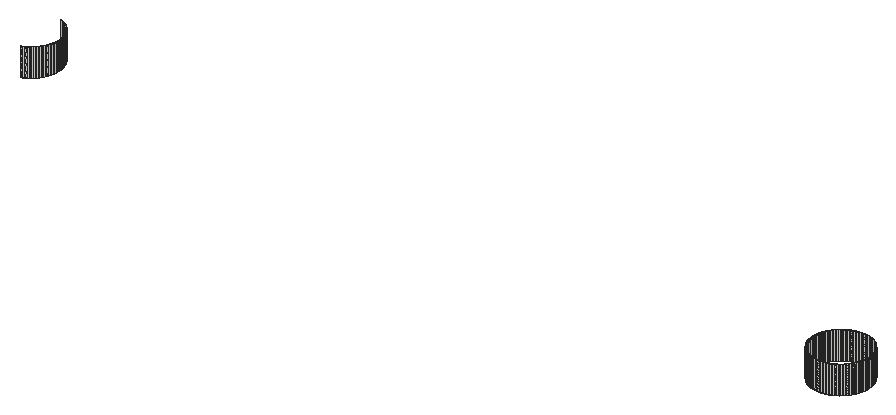
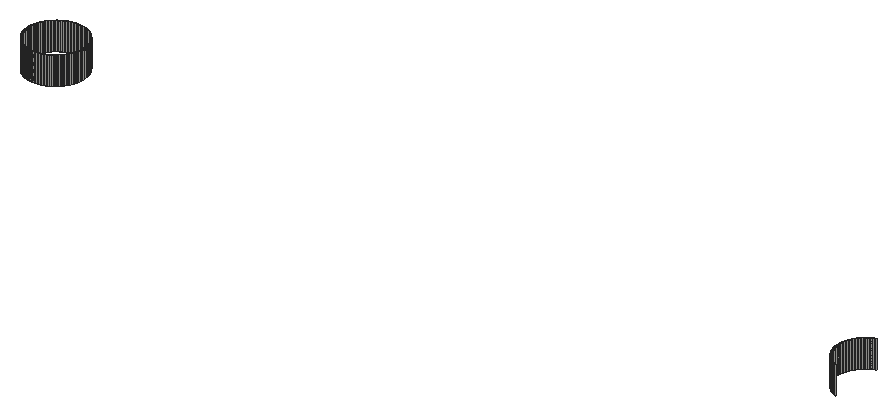
# SketchUp Ruby script. Lengths in inches.
U = 1.inch
M = Sketchup.active_model
def pt(a) = Geom::Point3d.new(a.map { |v| v * U })
def face(e, loops, mat)
  f = e.add_face(loops[0].map { |a| pt(a) })
  loops[1..].each { |l| e.add_face(l.map { |a| pt(a) }).erase! }
  f.material = f.back_material = mat if mat
  f
end
# faces: each face lists its corners as indices into pts; further lists are holes
def faces(e, pts, list, mat = nil) = list.each { |f| face(e, (f[0].is_a?(Array) ? f : [f]).map { |l| l.map { |i| pts[i] } }, mat) }
# xy, xz, yz: faces in a plane at the given z, y or x. An outline is a flat list of corners, or four numbers for a rectangle; further outlines are holes
def ring(l) = l.size == 4 ? [[l[0], l[1]], [l[2], l[1]], [l[2], l[3]], [l[0], l[3]]] : l.each_slice(2).to_a
def flat(e, list, mat, &to3) = list.each { |f| face(e, (f[0].is_a?(Array) ? f : [f]).map { |l| ring(l).map { |u, v| to3.(u, v) } }, mat) }
def xy(e, z, list, mat = nil) = flat(e, list, mat) { |x, y| [x, y, z] }
def xz(e, y, list, mat = nil) = flat(e, list, mat) { |x, z| [x, y, z] }
def yz(e, x, list, mat = nil) = flat(e, list, mat) { |y, z| [x, y, z] }
def lines(e, pts, list) = list.each { |a, b| e.add_line(pt(pts[a]), pt(pts[b])) }
# prism: a flat outline (further loops are holes) pulled along v
def prism(e, loops, v, mat = nil)
  f = face(e, loops, mat); d = Geom::Vector3d.new(v.map { |x| x * U })
  f.pushpull(f.normal.samedirection?(d) ? d.length : -d.length)
end
def box(e, o, s, mat = nil) = prism(e, [[o, [o[0] + s[0], o[1], o[2]], [o[0] + s[0], o[1] + s[1], o[2]], [o[0], o[1] + s[1], o[2]]]], [0, 0, s[2]], mat)
def at(x, y, z, deg = 0) = Geom::Transformation.translation(pt([x, y, z])) * Geom::Transformation.rotation(ORIGIN, Z_AXIS, deg.degrees)
def axes(o, x, y, z) = Geom::Transformation.new([*x, 0, *y, 0, *z, 0, *pt(o).to_a, 1])
def part(name) = M.definitions.add(name)
# library, detail: a bought-in or finely detailed component or shape, given as its bounding box
def library(name, o, s) = part(name).tap { |d| box(d.entities, o, s) }
def detail(e, o, s) = box(e.add_group.entities, o, s)
def put(e, d, t, mat = nil) = e.add_instance(d, t).tap { |i| i.material = mat if mat }
def group(e, t, mat = nil) = e.add_group.tap { |g| g.transformation = t; g.material = mat if mat }.entities
root = M.entities
xz(root,174.5,[[291.84,258,291.92,261],[291.92,258,292,261],[292,258,292.08,261],[292.08,258,292.16,261]])
xz(root,180.5,[[291.84,258,291.92,261],[291.92,258,292,261],[292,258,292.08,261],[292.08,258,292.16,261]])
yz(root,207.32,[[177.1875,258,177.26,261],[177.74,258,177.8125,261]])
yz(root,207.33,[[177.34,258,177.42,261],[177.42,258,177.5,261],[177.5,258,177.58,261],[177.58,258,177.66,261]])
yz(root,289,[[177.34,258,177.42,261],[177.42,258,177.5,261],[177.5,258,177.58,261],[177.58,258,177.66,261]])
yz(root,295,[[177.34,258,177.42,261],[177.42,258,177.5,261],[177.5,258,177.58,261],[177.58,258,177.66,261]])
p = [[291.53,174.54,258],[291.45,174.55,258],[291.45,174.55,261],[291.53,174.54,261],[291.61,174.53,258],[291.61,174.53,261],
  [291.6875,174.52,258],[291.6875,174.52,261],[291.76,174.51,258],[291.76,174.51,261],[291.84,174.5,258],[291.84,174.5,261],
  [292.24,174.51,258],[292.16,174.5,258],[292.16,174.5,261],[292.24,174.51,261],[292.3125,174.52,258],[292.3125,174.52,261],
  [292.39,174.53,258],[292.39,174.53,261],[292.47,174.54,258],[292.47,174.54,261],[292.55,174.55,258],[292.55,174.55,261],
  [291.07,174.65,258],[291,174.67,258],[291,174.67,261],[291.07,174.65,261],[291.15,174.625,258],[291.15,174.625,261],
  [291.22,174.6,258],[291.22,174.6,261],[291.3,174.58,258],[291.3,174.58,261],[291.375,174.57,258],[291.375,174.57,261],
  [292.625,174.57,258],[292.625,174.57,261],[292.7,174.58,258],[292.7,174.58,261],[292.78,174.6,258],[292.78,174.6,261],
  [292.85,174.625,258],[292.85,174.625,261],[292.93,174.65,258],[292.93,174.65,261],[293,174.67,258],[293,174.67,261],
  [205.48,174.73,258],[205.41,174.7,258],[205.41,174.7,261],[205.48,174.73,261],[205.55,174.76,258],[205.55,174.76,261],
  [290.85,174.73,258],[290.78,174.76,258],[290.78,174.76,261],[290.85,174.73,261],[290.92,174.7,258],[290.92,174.7,261],
  [293.08,174.7,258],[293.08,174.7,261],[293.15,174.73,258],[293.15,174.73,261],[293.22,174.76,258],[293.22,174.76,261],
  [205.625,174.79,258],[205.625,174.79,261],[205.7,174.83,258],[205.7,174.83,261],[205.76,174.86,258],[205.76,174.86,261],
  [290.64,174.83,258],[290.57,174.86,258],[290.57,174.86,261],[290.64,174.83,261],[290.71,174.79,258],[290.71,174.79,261],
  [293.29,174.79,258],[293.29,174.79,261],[293.36,174.83,258],[293.36,174.83,261],[293.43,174.86,258],[293.43,174.86,261],
  [205.83,174.9,258],[205.83,174.9,261],[205.9,174.94,258],[205.9,174.94,261],[205.97,174.98,258],[205.97,174.98,261],
  [290.43,174.94,258],[290.37,174.98,258],[290.37,174.98,261],[290.43,174.94,261],[290.5,174.9,258],[290.5,174.9,261],
  [293.5,174.9,258],[293.5,174.9,261],[293.57,174.94,258],[293.57,174.94,261],[293.63,174.98,258],[293.63,174.98,261],
  [206.03,175.03,258],[206.03,175.03,261],[206.1,175.07,258],[206.1,175.07,261],[290.3,175.03,258],[290.24,175.07,258],
  [290.24,175.07,261],[290.3,175.03,261],[293.7,175.03,258],[293.7,175.03,261],[293.76,175.07,258],[293.76,175.07,261],
  [206.16,175.12,258],[206.16,175.12,261],[206.22,175.17,258],[206.22,175.17,261],[290.17,175.12,258],[290.11,175.17,258],
  [290.11,175.17,261],[290.17,175.12,261],[293.83,175.12,258],[293.83,175.12,261],[293.89,175.17,258],[293.89,175.17,261],
  [206.28,175.22,258],[206.28,175.22,261],[206.34,175.27,258],[206.34,175.27,261],[290.05,175.22,258],[289.99,175.27,258],
  [289.99,175.27,261],[290.05,175.22,261],[293.95,175.22,258],[293.95,175.22,261],[294.01,175.27,258],[294.01,175.27,261],
  [206.4,175.32,258],[206.4,175.32,261],[206.45,175.38,258],[206.45,175.38,261],[289.93,175.32,258],[289.88,175.38,258],
  [289.88,175.38,261],[289.93,175.32,261],[294.07,175.32,258],[294.07,175.32,261],[294.12,175.38,258],[294.12,175.38,261],
  [206.51,175.43,258],[206.51,175.43,261],[206.5625,175.49,258],[206.5625,175.49,261],[289.82,175.43,258],[289.77,175.49,258],
  [289.77,175.49,261],[289.82,175.43,261],[294.18,175.43,258],[294.18,175.43,261],[294.23,175.49,258],[294.23,175.49,261],
  [206.61,175.55,258],[206.61,175.55,261],[289.72,175.55,258],[289.72,175.55,261],[294.28,175.55,258],[294.28,175.55,261],
  [206.66,175.61,258],[206.66,175.61,261],[206.71,175.67,258],[206.71,175.67,261],[289.67,175.61,258],[289.62,175.67,258],
  [289.62,175.67,261],[289.67,175.61,261],[294.33,175.61,258],[294.33,175.61,261],[294.38,175.67,258],[294.38,175.67,261],
  [206.76,175.74,258],[206.76,175.74,261],[206.81,175.8,258],[206.81,175.8,261],[289.57,175.74,258],[289.53,175.8,258],
  [289.53,175.8,261],[289.57,175.74,261],[294.43,175.74,258],[294.43,175.74,261],[294.47,175.8,258],[294.47,175.8,261],
  [206.85,175.87,258],[206.85,175.87,261],[289.48,175.87,258],[289.48,175.87,261],[294.52,175.87,258],[294.52,175.87,261],
  [206.89,175.93,258],[206.89,175.93,261],[206.93,176,258],[206.93,176,261],[289.44,175.93,258],[289.4,176,258],
  [289.4,176,261],[289.44,175.93,261],[294.56,175.93,258],[294.56,175.93,261],[294.6,176,258],[294.6,176,261],
  [206.97,176.07,258],[206.97,176.07,261],[289.36,176.07,258],[289.36,176.07,261],[294.64,176.07,258],[294.64,176.07,261],
  [207.01,176.14,258],[207.01,176.14,261],[207.04,176.21,258],[207.04,176.21,261],[289.33,176.14,258],[289.29,176.21,258],
  [289.29,176.21,261],[289.33,176.14,261],[294.67,176.14,258],[294.67,176.14,261],[294.71,176.21,258],[294.71,176.21,261],
  [207.07,176.28,258],[207.07,176.28,261],[289.26,176.28,258],[289.26,176.28,261],[294.74,176.28,258],[294.74,176.28,261],
  [207.1,176.35,258],[207.1,176.35,261],[289.23,176.35,258],[289.23,176.35,261],[294.77,176.35,258],[294.77,176.35,261],
  [207.13,176.42,258],[207.13,176.42,261],[207.16,176.5,258],[207.16,176.5,261],[289.2,176.42,258],[289.17,176.5,258],
  [289.17,176.5,261],[289.2,176.42,261],[294.8,176.42,258],[294.8,176.42,261],[294.83,176.5,258],[294.83,176.5,261],
  [207.1875,176.57,258],[207.1875,176.57,261],[289.15,176.57,258],[289.15,176.57,261],[294.85,176.57,258],[294.85,176.57,261],
  [207.21,176.65,258],[207.21,176.65,261],[207.23,176.72,258],[207.23,176.72,261],[289.125,176.65,258],[289.1,176.72,258],
  [289.1,176.72,261],[289.125,176.65,261],[294.875,176.65,258],[294.875,176.65,261],[294.9,176.72,258],[294.9,176.72,261],
  [207.25,176.8,258],[207.25,176.8,261],[289.08,176.8,258],[289.08,176.8,261],[294.92,176.8,258],[294.92,176.8,261],
  [207.27,176.875,258],[207.27,176.875,261],[289.07,176.875,258],[289.07,176.875,261],[294.93,176.875,258],[294.93,176.875,261],
  [207.28,176.95,258],[207.28,176.95,261],[289.05,176.95,258],[289.05,176.95,261],[294.95,176.95,258],[294.95,176.95,261],
  [207.3,177.03,258],[207.3,177.03,261],[207.31,177.11,258],[207.31,177.11,261],[289.04,177.03,258],[289.03,177.11,258],
  [289.03,177.11,261],[289.04,177.03,261],[294.96,177.03,258],[294.96,177.03,261],[294.97,177.11,258],[294.97,177.11,261],
  [207.32,177.1875,258],[207.32,177.1875,261],[289.02,177.1875,258],[289.02,177.1875,261],[294.98,177.1875,258],[294.98,177.1875,261],
  [289.01,177.26,258],[289.01,177.26,261],[294.99,177.26,258],[294.99,177.26,261],[207.33,177.34,258],[207.32,177.26,258],
  [207.32,177.26,261],[207.33,177.34,261],[289,177.34,258],[289,177.34,261],[295,177.34,258],[295,177.34,261],
  [207.32,177.74,258],[207.33,177.66,258],[207.33,177.66,261],[207.32,177.74,261],[289,177.66,258],[289.01,177.74,258],
  [289.01,177.74,261],[289,177.66,261],[289.02,177.8125,258],[289.02,177.8125,261],[294.98,177.8125,258],[294.99,177.74,258],
  [294.99,177.74,261],[294.98,177.8125,261],[295,177.66,258],[295,177.66,261],[207.31,177.89,258],[207.32,177.8125,258],
  [207.32,177.8125,261],[207.31,177.89,261],[289.03,177.89,258],[289.03,177.89,261],[294.97,177.89,258],[294.97,177.89,261],
  [207.3,177.97,258],[207.3,177.97,261],[289.04,177.97,258],[289.04,177.97,261],[294.96,177.97,258],[294.96,177.97,261],
  [207.27,178.125,258],[207.28,178.05,258],[207.28,178.05,261],[207.27,178.125,261],[289.05,178.05,258],[289.05,178.05,261],
  [289.07,178.125,258],[289.07,178.125,261],[294.93,178.125,258],[294.95,178.05,258],[294.95,178.05,261],[294.93,178.125,261],
  [207.25,178.2,258],[207.25,178.2,261],[289.08,178.2,258],[289.08,178.2,261],[294.92,178.2,258],[294.92,178.2,261],
  [207.23,178.28,258],[207.23,178.28,261],[289.1,178.28,258],[289.1,178.28,261],[294.9,178.28,258],[294.9,178.28,261],
  [207.21,178.35,258],[207.21,178.35,261],[289.125,178.35,258],[289.125,178.35,261],[294.875,178.35,258],[294.875,178.35,261],
  [207.16,178.5,258],[207.1875,178.43,258],[207.1875,178.43,261],[207.16,178.5,261],[289.15,178.43,258],[289.15,178.43,261],
  [289.17,178.5,258],[289.17,178.5,261],[294.83,178.5,258],[294.85,178.43,258],[294.85,178.43,261],[294.83,178.5,261],
  [207.13,178.58,258],[207.13,178.58,261],[289.2,178.58,258],[289.2,178.58,261],[294.8,178.58,258],[294.8,178.58,261],
  [207.07,178.72,258],[207.1,178.65,258],[207.1,178.65,261],[207.07,178.72,261],[289.23,178.65,258],[289.23,178.65,261],
  [289.26,178.72,258],[289.26,178.72,261],[294.74,178.72,258],[294.77,178.65,258],[294.77,178.65,261],[294.74,178.72,261],
  [207.04,178.79,258],[207.04,178.79,261],[289.29,178.79,258],[289.29,178.79,261],[294.71,178.79,258],[294.71,178.79,261],
  [207.01,178.86,258],[207.01,178.86,261],[289.33,178.86,258],[289.33,178.86,261],[294.67,178.86,258],[294.67,178.86,261],
  [206.93,179,258],[206.97,178.93,258],[206.97,178.93,261],[206.93,179,261],[289.36,178.93,258],[289.36,178.93,261],
  [289.4,179,258],[289.4,179,261],[294.6,179,258],[294.64,178.93,258],[294.64,178.93,261],[294.6,179,261],
  [206.89,179.07,258],[206.89,179.07,261],[289.44,179.07,258],[289.44,179.07,261],[294.56,179.07,258],[294.56,179.07,261],
  [206.81,179.2,258],[206.85,179.13,258],[206.85,179.13,261],[206.81,179.2,261],[289.48,179.13,258],[289.48,179.13,261],
  [289.53,179.2,258],[289.53,179.2,261],[294.47,179.2,258],[294.52,179.13,258],[294.52,179.13,261],[294.47,179.2,261],
  [206.76,179.26,258],[206.76,179.26,261],[289.57,179.26,258],[289.57,179.26,261],[294.43,179.26,258],[294.43,179.26,261],
  [206.66,179.39,258],[206.71,179.33,258],[206.71,179.33,261],[206.66,179.39,261],[289.62,179.33,258],[289.62,179.33,261],
  [289.67,179.39,258],[289.67,179.39,261],[294.33,179.39,258],[294.38,179.33,258],[294.38,179.33,261],[294.33,179.39,261],
  [206.5625,179.51,258],[206.61,179.45,258],[206.61,179.45,261],[206.5625,179.51,261],[289.72,179.45,258],[289.72,179.45,261],
  [289.77,179.51,258],[289.77,179.51,261],[294.23,179.51,258],[294.28,179.45,258],[294.28,179.45,261],[294.23,179.51,261],
  [206.51,179.57,258],[206.51,179.57,261],[289.82,179.57,258],[289.82,179.57,261],[294.18,179.57,258],[294.18,179.57,261],
  [206.4,179.68,258],[206.45,179.62,258],[206.45,179.62,261],[206.4,179.68,261],[289.88,179.62,258],[289.88,179.62,261],
  [289.93,179.68,258],[289.93,179.68,261],[294.07,179.68,258],[294.12,179.62,258],[294.12,179.62,261],[294.07,179.68,261],
  [206.28,179.78,258],[206.34,179.73,258],[206.34,179.73,261],[206.28,179.78,261],[289.99,179.73,258],[289.99,179.73,261],
  [290.05,179.78,258],[290.05,179.78,261],[293.95,179.78,258],[294.01,179.73,258],[294.01,179.73,261],[293.95,179.78,261],
  [206.16,179.88,258],[206.22,179.83,258],[206.22,179.83,261],[206.16,179.88,261],[290.11,179.83,258],[290.11,179.83,261],
  [290.17,179.88,258],[290.17,179.88,261],[293.83,179.88,258],[293.89,179.83,258],[293.89,179.83,261],[293.83,179.88,261],
  [206.03,179.97,258],[206.1,179.93,258],[206.1,179.93,261],[206.03,179.97,261],[290.24,179.93,258],[290.24,179.93,261],
  [290.3,179.97,258],[290.3,179.97,261],[293.7,179.97,258],[293.76,179.93,258],[293.76,179.93,261],[293.7,179.97,261],
  [205.9,180.06,258],[205.97,180.02,258],[205.97,180.02,261],[205.9,180.06,261],[290.37,180.02,258],[290.37,180.02,261],
  [290.43,180.06,258],[290.43,180.06,261],[293.57,180.06,258],[293.63,180.02,258],[293.63,180.02,261],[293.57,180.06,261],
  [205.7,180.17,258],[205.76,180.14,258],[205.76,180.14,261],[205.7,180.17,261],[205.83,180.1,258],[205.83,180.1,261],
  [290.5,180.1,258],[290.5,180.1,261],[290.57,180.14,258],[290.57,180.14,261],[290.64,180.17,258],[290.64,180.17,261],
  [293.36,180.17,258],[293.43,180.14,258],[293.43,180.14,261],[293.36,180.17,261],[293.5,180.1,258],[293.5,180.1,261],
  [205.48,180.27,258],[205.55,180.24,258],[205.55,180.24,261],[205.48,180.27,261],[205.625,180.21,258],[205.625,180.21,261],
  [290.71,180.21,258],[290.71,180.21,261],[290.78,180.24,258],[290.78,180.24,261],[290.85,180.27,258],[290.85,180.27,261],
  [293.15,180.27,258],[293.22,180.24,258],[293.22,180.24,261],[293.15,180.27,261],[293.29,180.21,258],[293.29,180.21,261],
  [205.33,180.33,258],[205.41,180.3,258],[205.41,180.3,261],[205.33,180.33,261],[290.92,180.3,258],[290.92,180.3,261],
  [291,180.33,258],[291,180.33,261],[291.07,180.35,258],[291.07,180.35,261],[292.93,180.35,258],[293,180.33,258],
  [293,180.33,261],[292.93,180.35,261],[293.08,180.3,258],[293.08,180.3,261],[291.15,180.375,258],[291.15,180.375,261],
  [291.22,180.4,258],[291.22,180.4,261],[291.3,180.42,258],[291.3,180.42,261],[291.375,180.43,258],[291.375,180.43,261],
  [291.45,180.45,258],[291.45,180.45,261],[291.53,180.46,258],[291.53,180.46,261],[292.47,180.46,258],[292.55,180.45,258],
  [292.55,180.45,261],[292.47,180.46,261],[292.625,180.43,258],[292.625,180.43,261],[292.7,180.42,258],[292.7,180.42,261],
  [292.78,180.4,258],[292.78,180.4,261],[292.85,180.375,258],[292.85,180.375,261],[291.61,180.47,258],[291.61,180.47,261],
  [291.6875,180.48,258],[291.6875,180.48,261],[291.76,180.49,258],[291.76,180.49,261],[291.84,180.5,258],[291.84,180.5,261],
  [292.16,180.5,258],[292.24,180.49,258],[292.24,180.49,261],[292.16,180.5,261],[292.3125,180.48,258],[292.3125,180.48,261],
  [292.39,180.47,258],[292.39,180.47,261]]
faces(root,p,[[0,1,2,3],[4,0,3,5],[6,4,5,7],[8,6,7,9],[10,8,9,11],[12,13,14,15],[16,12,15,17],[18,16,17,19],
  [20,18,19,21],[22,20,21,23],[24,25,26,27],[28,24,27,29],[30,28,29,31],[32,30,31,33],[34,32,33,35],[1,34,35,2],
  [36,22,23,37],[38,36,37,39],[40,38,39,41],[42,40,41,43],[44,42,43,45],[46,44,45,47],[48,49,50,51],[52,48,51,53],
  [54,55,56,57],[58,54,57,59],[25,58,59,26],[60,46,47,61],[62,60,61,63],[64,62,63,65],[66,52,53,67],[68,66,67,69],
  [70,68,69,71],[72,73,74,75],[76,72,75,77],[55,76,77,56],[78,64,65,79],[80,78,79,81],[82,80,81,83],[84,70,71,85],
  [86,84,85,87],[88,86,87,89],[90,91,92,93],[94,90,93,95],[73,94,95,74],[96,82,83,97],[98,96,97,99],[100,98,99,101],
  [102,88,89,103],[104,102,103,105],[106,107,108,109],[91,106,109,92],[110,100,101,111],[112,110,111,113],[114,104,105,115],[116,114,115,117],
  [118,119,120,121],[107,118,121,108],[122,112,113,123],[124,122,123,125],[126,116,117,127],[128,126,127,129],[130,131,132,133],[119,130,133,120],
  [134,124,125,135],[136,134,135,137],[138,128,129,139],[140,138,139,141],[142,143,144,145],[131,142,145,132],[146,136,137,147],[148,146,147,149],
  [150,140,141,151],[152,150,151,153],[154,155,156,157],[143,154,157,144],[158,148,149,159],[160,158,159,161],[162,152,153,163],[155,164,165,156],
  [166,160,161,167],[168,162,163,169],[170,168,169,171],[172,173,174,175],[164,172,175,165],[176,166,167,177],[178,176,177,179],[180,170,171,181],
  [182,180,181,183],[184,185,186,187],[173,184,187,174],[188,178,179,189],[190,188,189,191],[192,182,183,193],[185,194,195,186],[196,190,191,197],
  [198,192,193,199],[200,198,199,201],[202,203,204,205],[194,202,205,195],[206,196,197,207],[208,206,207,209],[210,200,201,211],[203,212,213,204],
  [214,208,209,215],[216,210,211,217],[218,216,217,219],[220,221,222,223],[212,220,223,213],[224,214,215,225],[226,224,225,227],[228,218,219,229],
  [221,230,231,222],[232,226,227,233],[234,228,229,235],[230,236,237,231],[238,232,233,239],[240,234,235,241],[242,240,241,243],[244,245,246,247],
  [236,244,247,237],[248,238,239,249],[250,248,249,251],[252,242,243,253],[245,254,255,246],[256,250,251,257],[258,252,253,259],[260,258,259,261],
  [262,263,264,265],[254,262,265,255],[266,256,257,267],[268,266,267,269],[270,260,261,271],[263,272,273,264],[274,268,269,275],[276,270,271,277],
  [272,278,279,273],[280,274,275,281],[282,276,277,283],[278,284,285,279],[286,280,281,287],[288,282,283,289],[290,288,289,291],[292,293,294,295],
  [284,292,295,285],[296,286,287,297],[298,296,297,299],[300,290,291,301],[293,302,303,294],[304,298,299,305],[302,306,307,303],[308,304,305,309],
  [310,311,312,313],[306,314,315,307],[316,308,309,317],[318,319,320,321],[322,323,324,325],[323,326,327,324],[328,329,330,331],[329,332,333,330],
  [334,335,336,337],[326,338,339,327],[340,328,331,341],[342,334,337,343],[338,344,345,339],[346,340,341,347],[348,349,350,351],[349,342,343,350],
  [344,352,353,345],[352,354,355,353],[356,357,358,359],[357,346,347,358],[360,348,351,361],[354,362,363,355],[364,356,359,365],[366,360,361,367],
  [362,368,369,363],[370,364,365,371],[372,366,367,373],[368,374,375,369],[376,370,371,377],[378,379,380,381],[379,372,373,380],[374,382,383,375],
  [382,384,385,383],[386,387,388,389],[387,376,377,388],[390,378,381,391],[384,392,393,385],[394,386,389,395],[396,397,398,399],[397,390,391,398],
  [392,400,401,393],[400,402,403,401],[404,405,406,407],[405,394,395,406],[408,396,399,409],[402,410,411,403],[412,404,407,413],[414,408,409,415],
  [410,416,417,411],[418,412,413,419],[420,421,422,423],[421,414,415,422],[416,424,425,417],[424,426,427,425],[428,429,430,431],[429,418,419,430],
  [432,420,423,433],[426,434,435,427],[436,428,431,437],[438,439,440,441],[439,432,433,440],[434,442,443,435],[442,444,445,443],[446,447,448,449],
  [447,436,437,448],[450,438,441,451],[444,452,453,445],[454,446,449,455],[456,457,458,459],[457,450,451,458],[452,460,461,453],[460,462,463,461],
  [464,465,466,467],[465,454,455,466],[468,469,470,471],[469,456,459,470],[462,472,473,463],[472,474,475,473],[476,477,478,479],[477,464,467,478],
  [480,468,471,481],[474,482,483,475],[484,476,479,485],[486,487,488,489],[487,480,481,488],[482,490,491,483],[490,492,493,491],[494,495,496,497],
  [495,484,485,496],[498,499,500,501],[499,486,489,500],[492,502,503,493],[502,504,505,503],[506,507,508,509],[507,494,497,508],[510,511,512,513],
  [511,498,501,512],[504,514,515,505],[514,516,517,515],[518,519,520,521],[519,506,509,520],[522,523,524,525],[523,510,513,524],[516,526,527,517],
  [526,528,529,527],[530,531,532,533],[531,518,521,532],[534,535,536,537],[535,522,525,536],[528,538,539,529],[538,540,541,539],[542,543,544,545],
  [543,530,533,544],[546,547,548,549],[547,550,551,548],[550,534,537,551],[540,552,553,541],[552,554,555,553],[554,556,557,555],[558,559,560,561],
  [559,562,563,560],[562,542,545,563],[564,565,566,567],[565,568,569,566],[568,546,549,569],[556,570,571,557],[570,572,573,571],[572,574,575,573],
  [576,577,578,579],[577,580,581,578],[580,558,561,581],[582,583,584,585],[583,564,567,584],[574,586,587,575],[586,588,589,587],[588,590,591,589],
  [592,593,594,595],[593,596,597,594],[596,576,579,597],[590,598,599,591],[598,600,601,599],[600,602,603,601],[602,604,605,603],[604,606,607,605],
  [606,608,609,607],[610,611,612,613],[611,614,615,612],[614,616,617,615],[616,618,619,617],[618,620,621,619],[620,592,595,621],[608,622,623,609],
  [622,624,625,623],[624,626,627,625],[626,628,629,627],[630,631,632,633],[631,634,635,632],[634,636,637,635],[636,610,613,637]])
